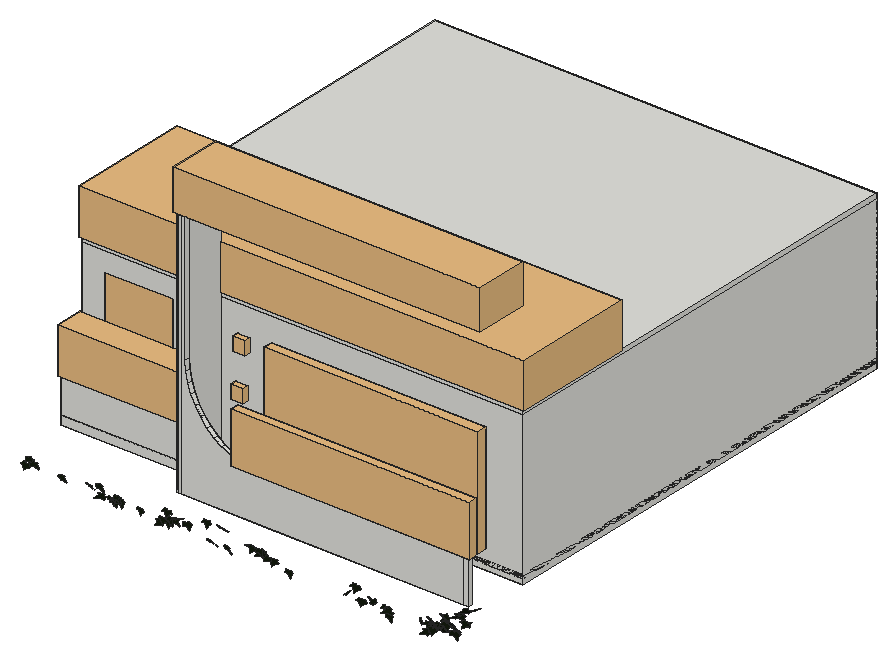
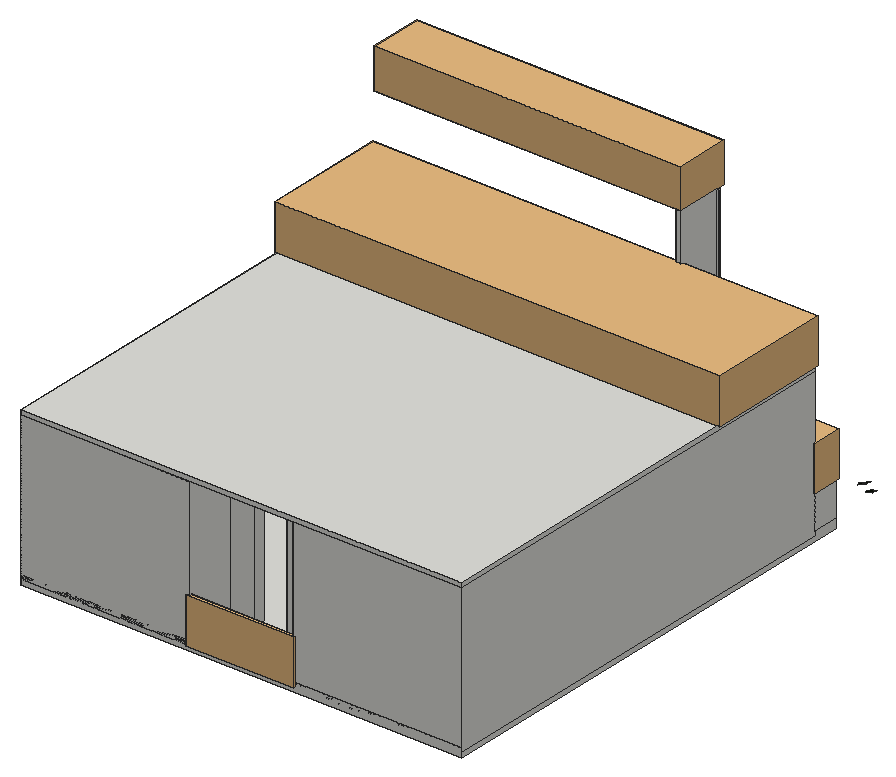
# SketchUp Ruby script. Lengths in millimetres.
U = 1.mm
M = Sketchup.active_model
def pt(a) = Geom::Point3d.new(a.map { |v| v * U })
def face(e, loops, mat)
  f = e.add_face(loops[0].map { |a| pt(a) })
  loops[1..].each { |l| e.add_face(l.map { |a| pt(a) }).erase! }
  f.material = f.back_material = mat if mat
  f
end
# faces: each face lists its corners as indices into pts; further lists are holes
def faces(e, pts, list, mat = nil) = list.each { |f| face(e, (f[0].is_a?(Array) ? f : [f]).map { |l| l.map { |i| pts[i] } }, mat) }
# xy, xz, yz: faces in a plane at the given z, y or x. An outline is a flat list of corners, or four numbers for a rectangle; further outlines are holes
def ring(l) = l.size == 4 ? [[l[0], l[1]], [l[2], l[1]], [l[2], l[3]], [l[0], l[3]]] : l.each_slice(2).to_a
def flat(e, list, mat, &to3) = list.each { |f| face(e, (f[0].is_a?(Array) ? f : [f]).map { |l| ring(l).map { |u, v| to3.(u, v) } }, mat) }
def xy(e, z, list, mat = nil) = flat(e, list, mat) { |x, y| [x, y, z] }
def xz(e, y, list, mat = nil) = flat(e, list, mat) { |x, z| [x, y, z] }
def yz(e, x, list, mat = nil) = flat(e, list, mat) { |y, z| [x, y, z] }
def lines(e, pts, list) = list.each { |a, b| e.add_line(pt(pts[a]), pt(pts[b])) }
# prism: a flat outline (further loops are holes) pulled along v
def prism(e, loops, v, mat = nil)
  f = face(e, loops, mat); d = Geom::Vector3d.new(v.map { |x| x * U })
  f.pushpull(f.normal.samedirection?(d) ? d.length : -d.length)
end
def box(e, o, s, mat = nil) = prism(e, [[o, [o[0] + s[0], o[1], o[2]], [o[0] + s[0], o[1] + s[1], o[2]], [o[0], o[1] + s[1], o[2]]]], [0, 0, s[2]], mat)
def at(x, y, z, deg = 0) = Geom::Transformation.translation(pt([x, y, z])) * Geom::Transformation.rotation(ORIGIN, Z_AXIS, deg.degrees)
def axes(o, x, y, z) = Geom::Transformation.new([*x, 0, *y, 0, *z, 0, *pt(o).to_a, 1])
def part(name) = M.definitions.add(name)
# library, detail: a bought-in or finely detailed component or shape, given as its bounding box
def library(name, o, s) = part(name).tap { |d| box(d.entities, o, s) }
def detail(e, o, s) = box(e.add_group.entities, o, s)
def put(e, d, t, mat = nil) = e.add_instance(d, t).tap { |i| i.material = mat if mat }
def group(e, t, mat = nil) = e.add_group.tap { |g| g.transformation = t; g.material = mat if mat }.entities
root = M.entities
M.materials.add("Emissive\#2").color = [255, 185, 108]
M.materials.add("efeu1").color = [18, 25, 13]
c1 = part("ivyleaf_9")
p = [[39.1,54.8,31.7],[34.5,51.8,30.2],[-5.3,25.2,17.3],[-17.9,28.3,20.9],[-21.6,21.7,17],[-20.2,4.3,5.3],
  [-22.9,-0.3,2.5],[-17.1,-4,-0.6],[-2,-2.1,-1.2],[-0.7,-15.4,-10.1],[16.6,-22.3,-16.7],[21.1,-15.1,-12.5],
  [32.7,-10.7,-11],[46.1,-1.8,-6.6],[30.8,11.2,3.8]]
faces(c1.entities,p,[[0,1,2,3,4,5,6,7,8,9,10,11,12,13,14]],"efeu1")
c2 = part("Group\#8")
g1 = group(c2.entities,at(0,0,0))
xy(g1,0,[[0,0,0,9144,3500.3,9144,3500.3,8102.6,4459.1,8102.6,4459.1,7874,3276.6,7874,3276.6,8915.4,228.6,8915.4,228.6,228.6,8915.4,228.6,8915.4,8915.4,5867.4,8915.4,5867.4,7874,5119.1,7874,5119.1,8102.6,5638.8,8102.6,5638.8,9144,9144,9144,9144,0]])
xy(g1,288,[[3929.6,0,8374.6,228.6],[4394.2,228.6,4521.2,579.4]])
xy(g1,376.3,[[475.3,0,1877,723.9]])
xy(g1,2564.5,[[3929.6,0,8374.6,228.6],[4394.2,228.6,4521.2,579.4]])
xy(g1,2644.4,[[475.3,0,1877,723.9]])
xy(g1,3048,[[0,0,9144,0,9144,9144,5638.8,9144,5638.8,8102.6,5119.1,8102.6,5119.1,7874,5867.4,7874,5867.4,8915.4,8915.4,8915.4,8915.4,228.6,228.6,228.6,228.6,8915.4,3276.6,8915.4,3276.6,7874,4459.1,7874,4459.1,8102.6,3500.3,8102.6,3500.3,9144,0,9144]])
xz(g1,0,[[[0,0,9144,3048],[3929.6,288,8374.6,2564.5],[475.3,376.3,1877,2644.4]]])
xz(g1,228.6,[[1447.8,0,1574.8,3048],[4394.2,0,4521.2,288],[4521.2,0,4521.2,288,8374.6,288,8374.6,2564.5,4521.2,2564.5,4521.2,3048,8915.4,3048,8915.4,0],[3929.6,288,4394.2,2564.5],[4394.2,2564.5,4521.2,3048]])
xz(g1,579.4,[[4394.2,288,4521.2,2564.5]])
xz(g1,723.9,[[475.3,376.3,1877,2644.4]])
xz(g1,7874,[[3276.6,0,3403.6,3048],[3403.6,0,4459.1,3048],[5119.1,0,5740.4,3048],[5740.4,0,5867.4,3048]])
xz(g1,8102.6,[[3500.3,0,4459.1,3048],[5119.1,0,5638.8,3048]])
xz(g1,8915.4,[[228.6,0,3276.6,3048],[5867.4,0,8915.4,3048]])
xz(g1,9144,[[0,0,3500.3,3048],[5638.8,0,9144,3048]])
yz(g1,0,[[0,0,9144,3048]])
yz(g1,228.6,[[228.6,0,2362.2,3048],[2362.2,0,2489.2,3048],[2489.2,0,5334,3048],[5334,0,5461,3048],[5461,0,8915.4,3048]])
yz(g1,475.3,[[0,376.3,723.9,2644.4]])
yz(g1,1877,[[0,376.3,723.9,2644.4]])
yz(g1,3276.6,[[7874,0,8915.4,3048]])
yz(g1,3500.3,[[8102.6,0,9144,3048]])
yz(g1,3929.6,[[0,288,228.6,2564.5]])
yz(g1,4394.2,[[228.6,288,579.4,2564.5]])
yz(g1,4459.1,[[7874,0,8102.6,3048]])
yz(g1,4521.2,[[228.6,288,579.4,2564.5]])
yz(g1,5119.1,[[7874,0,8102.6,3048]])
yz(g1,5638.8,[[8102.6,0,9144,3048]])
yz(g1,5867.4,[[7874,0,8915.4,3048]])
yz(g1,8374.6,[[0,288,228.6,2564.5]])
yz(g1,8915.4,[[228.6,0,5334,3048],[5334,0,5461,3048],[5461,0,8915.4,3048]])
yz(g1,9144,[[0,0,9144,3048]])
c3 = library("Group\#24",[0,0,0],[2238.5,80,939.4])
c4 = library("EP Casement KUN43",[213.5,133.1,19],[2173.1,999.9,208])
c5 = library("ITDHP",[-33.4,-34.2,-15.9],[968.5,150,1668.6])
c6 = library("Group\#17",[0,0,0],[2782,637.9,939.4])
c7 = library("Group\#26",[0,0,0],[4943.1,178,1057.4])
c8 = library("Spot Light\#2",[-129.6,-129.6,-280.7],[259.2,259.2,280.7])
c9 = part("Group263\#1")
p = [[0,0,0],[0,0,-885.4],[-221.6,0,-885.4],[1442.9,-1423.4,0],[-1442.9,-1423.4,0],[1442.9,1423.4,0],
  [1442.9,0,0],[-1442.9,1423.4,0],[221.6,0,-885.4],[-1442.9,0,0],[0,0,-1433.1]]
lines(c9.entities,p,[[0,1],[1,2],[3,4],[5,6],[7,5],[1,8],[9,0],[0,6],[8,10],[4,9],[6,3],[2,10],
  [9,7]])
c10 = part("Rectangle Light\#7")
put(c10.entities,c9,at(0,0,0))
c11 = library("Spot Light\#1",[-129.6,-129.6,-280.7],[259.2,259.2,280.7])
c12 = part("Group265\#1")
p = [[0,0,0],[0,0,-130.3],[-40.5,0,-130.3],[263.6,-158.2,0],[-263.6,-158.2,0],[263.6,158.2,0],
  [263.6,0,0],[-263.6,158.2,0],[40.5,0,-130.3],[-263.6,0,0],[0,0,-210.9]]
lines(c12.entities,p,[[0,1],[1,2],[3,4],[5,6],[7,5],[1,8],[9,0],[0,6],[8,10],[4,9],[6,3],[2,10],
  [9,7]])
c13 = part("Rectangle Light\#8")
put(c13.entities,c12,at(0,0,0))
c14 = part("Group267\#1")
p = [[0,0,0],[0,0,-108.5],[-7.2,0,-108.5],[46.9,-304.4,0],[-46.9,-304.4,0],[46.9,304.4,0],
  [46.9,0,0],[-46.9,304.4,0],[7.2,0,-108.5],[-46.9,0,0],[0,0,-175.7]]
lines(c14.entities,p,[[0,1],[1,2],[3,4],[5,6],[7,5],[1,8],[9,0],[0,6],[8,10],[4,9],[6,3],[2,10],
  [9,7]])
c15 = part("Rectangle Light\#9")
put(c15.entities,c14,at(0,0,0))
c16 = part("Group\#23")
box(c16.entities,[0,0,0],[9144,9144,101.6])
c17 = library("Group\#22",[0,0,0],[9224,2553.9,939.4])
c18 = library("Group\#21",[0,0,0],[6357.6,1104,823.9])
put(root,c1,axes([5592.3,460.8,6161.6],[2.45685,-0.59225,0.48479],[0.84867,-0.19058,-1.42023],[1.18387,1.3657,0.01204]))
put(root,c1,axes([4619,464.9,6158.3],[-2.79662,0.20864,-0.05049],[0.09953,0.00914,-1.48408],[-0.39623,-1.47027,-0.01639]))
put(root,c1,axes([10268,425.7,6170.1],[-1.4631,-1.24601,-0.25563],[0.22649,0.22692,-1.46397],[2.41017,-0.77771,-0.01761]))
put(root,c1,axes([7263.1,462.9,6167.7],[-0.14093,-1.51309,0.00427],[-0.04602,-0.00309,-1.51471],[2.87935,-0.07411,-0.024]))
put(root,c1,axes([4716.1,516.7,6171.9],[-0.7949,-1.4134,0.1654],[0.47802,-0.24289,-1.44133],[2.66582,-0.3779,0.30777]))
put(root,c1,axes([10372.8,511.1,6164.8],[1.65053,-0.29109,1.18272],[2.16594,-0.32374,-0.91416],[0.82609,1.43043,0.03378]))
put(root,c1,axes([10269.6,291.9,6174.6],[-2.74592,0.3863,0.12497],[-0.24273,0.00675,-1.49338],[-0.73361,-1.44818,0.02637]))
put(root,c1,axes([3627.4,500.3,6194.9],[-1.06639,-1.24057,-0.64669],[0.46448,0.59927,-1.36106],[2.62177,-0.61076,-0.02191]))
put(root,c1,axes([8473.7,494.3,6187.5],[-1.19113,1.32112,-0.36173],[0.25067,-0.33782,-1.46166],[-2.59482,-0.63908,0.02485]))
put(root,c1,axes([9436.4,340.7,6172.9],[0.14762,-1.48528,-0.01857],[-0.00283,0.01852,-1.4873],[2.827,0.07758,-0.00052]))
put(root,c1,axes([8823.4,415.7,6193.8],[-2.34891,-0.65133,-0.55971],[1.00163,0.20073,-1.39408],[1.29154,-1.34023,0.06322]))
put(root,c1,axes([1750.2,554.6,6179.2],[-1.73355,-1.13881,0.03125],[-0.03879,-0.02372,-1.45827],[2.16785,-0.91109,-0.0011]))
put(root,c1,axes([10180.6,478.7,6189.5],[2.52486,-0.3914,0.50724],[1.00699,0.01154,-1.37491],[0.68762,1.42026,0.15096]))
put(root,c1,axes([10669.4,492.6,6209.1],[-1.53123,-0.68677,-1.08449],[1.55876,0.71089,-1.05779],[1.88117,-1.14807,-0.00625]))
put(root,c1,axes([9258.6,483.9,6194.2],[-0.71663,-1.45468,-0.11155],[0.03481,0.11049,-1.50259],[2.77646,-0.37685,-0.00995]))
put(root,c1,axes([6901.1,527.6,6212.4],[-2.33936,-0.72135,-0.37924],[0.61848,0.19554,-1.4252],[1.4224,-1.2714,-0.00403]))
put(root,c1,axes([10275.7,523.5,6224],[1.15166,-1.06105,-0.84161],[-0.7576,0.74174,-1.22134],[2.46366,0.72409,0.01784]))
put(root,c1,axes([9997.1,453.2,6220.6],[1.22078,-0.32697,-1.31555],[-1.94024,0.8429,-0.70657],[1.70043,1.19651,0.13825]))
put(root,c1,axes([10372.5,513.3,6206.3],[-1.98775,1.05541,-0.06008],[0.05793,-0.0544,-1.48474],[-2.01108,-1.04474,0.01661]))
put(root,c1,axes([3561.3,487.2,6213.5],[0.11986,-1.46571,0.35331],[0.14084,-0.35019,-1.46594],[2.86597,0.07851,0.05726]))
put(root,c1,axes([10155.9,478.2,6205.5],[-1.17879,-1.33704,0.0176],[-0.02173,-0.0141,-1.47353],[2.54479,-0.61946,-0.00443]))
put(root,c1,axes([3736.6,494.1,6224.2],[-0.60958,-1.40382,-0.44375],[0.24382,0.42583,-1.4396],[2.79142,-0.34376,0.02884]))
put(root,c1,axes([2486.8,523.6,6229],[1.16186,-1.22558,-0.56432],[-0.00212,0.61894,-1.3454],[2.56791,0.55503,0.25422]))
put(root,c1,axes([4161.4,487.7,6217.2],[-0.35936,-1.3491,0.65494],[0.1835,-0.66966,-1.35163],[2.84826,-0.12707,0.16971]))
put(root,c1,axes([4630.4,482.4,6217.6],[-0.54586,-1.41103,0.41049],[0.0843,-0.42634,-1.43459],[2.79554,-0.26266,0.12341]))
put(root,c1,axes([6025.6,392.6,6215.5],[1.17613,-1.38471,0.05444],[0.03392,-0.05166,-1.51634],[2.63719,0.61822,-0.00478]))
put(root,c1,axes([9008.2,469.4,6194.5],[-0.34678,0.4928,1.41934],[-1.29932,1.24646,-0.52041],[-2.54723,-0.7029,0.07223]))
put(root,c1,axes([10409.4,951,6249.6],[-0.83955,-0.7574,-1.2019],[1.7959,0.78456,-0.84074],[2.02115,-1.01174,0.2478]))
put(root,c1,axes([6789.8,499.5,6240.5],[-1.69721,-0.94294,0.75948],[-0.06872,-0.92212,-1.18726],[2.30329,-0.72233,0.52421]))
put(root,c1,axes([9453.6,348.6,6241.1],[-2.38252,-0.35015,0.73544],[-1.15559,-0.49772,-1.27051],[1.03335,-1.36391,0.27483]))
put(root,c1,axes([4789.2,504.7,6251.5],[-0.70683,-1.42641,-0.28886],[0.04876,0.29167,-1.47319],[2.76942,-0.36919,-0.04779]))
put(root,c1,axes([1890.8,531.5,6266.3],[0.35247,-1.18685,-0.84705],[0.73603,0.86326,-1.125],[2.6757,-0.08112,0.42105]))
put(root,c1,axes([4809.8,510.3,6251.9],[-1.89205,-1.10921,0.08797],[0.2323,-0.22597,-1.46984],[2.1049,-0.97211,0.24129]))
put(root,c1,axes([3467.3,391.1,6258.1],[-2.76338,-0.00649,0.40098],[-0.76319,0.04278,-1.45134],[-0.00978,-1.50571,-0.04296]))
put(root,c1,axes([10436.3,963.2,6256.3],[-0.01243,1.47025,0.19647],[-0.16686,0.19574,-1.46774],[-2.81811,-0.01808,0.08604]))
put(root,c1,axes([4872,497.4,6274.7],[0.54961,-1.3483,-0.57095],[0.00487,0.58241,-1.37407],[2.78666,0.26491,0.11501]))
put(root,c1,axes([3669.7,492.1,6272.8],[0.37008,-1.48559,-0.22501],[0.23777,0.24209,-1.49037],[2.84971,0.17273,0.15357]))
g2 = group(root,at(1385.3,2446,6197.6))
xy(g2,0,[[[1.6,-547.9,1.6,9144,9144,9144,9144,0,2496.5,0,2496.5,-547.9],[313.2,-413.3,353.1,-408,390.2,-392.6,422.1,-368.2,446.6,-336.3,462,-299.1,467.2,-259.3,462,-219.4,446.6,-182.3,422.1,-150.4,390.2,-125.9,353.1,-110.5,313.2,-105.3,273.4,-110.5,236.2,-125.9,204.3,-150.4,179.9,-182.3,164.5,-219.4,159.2,-259.3,164.5,-299.1,179.9,-336.3,204.3,-368.2,236.2,-392.6,273.4,-408],[1249,-413.3,1288.9,-408,1326,-392.6,1357.9,-368.2,1382.4,-336.3,1397.8,-299.1,1403,-259.3,1397.8,-219.4,1382.4,-182.3,1357.9,-150.4,1326,-125.9,1288.9,-110.5,1249,-105.3,1209.2,-110.5,1172.1,-125.9,1140.2,-150.4,1115.7,-182.3,1100.3,-219.4,1095.1,-259.3,1100.3,-299.1,1115.7,-336.3,1140.2,-368.2,1172.1,-392.6,1209.2,-408],[2184.9,-413.3,2224.7,-408,2261.9,-392.6,2293.8,-368.2,2318.2,-336.3,2333.6,-299.1,2338.9,-259.3,2333.6,-219.4,2318.2,-182.3,2293.8,-150.4,2261.9,-125.9,2224.7,-110.5,2184.9,-105.3,2145,-110.5,2107.9,-125.9,2076,-150.4,2051.5,-182.3,2036.1,-219.4,2030.9,-259.3,2036.1,-299.1,2051.5,-336.3,2076,-368.2,2107.9,-392.6,2145,-408]],[[313.2,-413.3,273.4,-408,236.2,-392.6,204.3,-368.2,179.9,-336.3,164.5,-299.1,159.2,-259.3,164.5,-219.4,179.9,-182.3,204.3,-150.4,236.2,-125.9,273.4,-110.5,313.2,-105.3,353.1,-110.5,390.2,-125.9,422.1,-150.4,446.6,-182.3,462,-219.4,467.2,-259.3,462,-299.1,446.6,-336.3,422.1,-368.2,390.2,-392.6,353.1,-408],[313.2,-357.7,338.7,-354.4,362.4,-344.5,382.8,-328.9,398.5,-308.5,408.3,-284.8,411.6,-259.3,408.3,-233.8,398.5,-210.1,382.8,-189.7,362.4,-174,338.7,-164.2,313.2,-160.9,287.7,-164.2,264,-174,243.6,-189.7,228,-210.1,218.1,-233.8,214.8,-259.3,218.1,-284.8,228,-308.5,243.6,-328.9,264,-344.5,287.7,-354.4]],[[1249,-413.3,1209.2,-408,1172.1,-392.6,1140.2,-368.2,1115.7,-336.3,1100.3,-299.1,1095.1,-259.3,1100.3,-219.4,1115.7,-182.3,1140.2,-150.4,1172.1,-125.9,1209.2,-110.5,1249,-105.3,1288.9,-110.5,1326,-125.9,1357.9,-150.4,1382.4,-182.3,1397.8,-219.4,1403,-259.3,1397.8,-299.1,1382.4,-336.3,1357.9,-368.2,1326,-392.6,1288.9,-408],[1249,-357.7,1274.5,-354.4,1298.3,-344.5,1318.6,-328.9,1334.3,-308.5,1344.1,-284.8,1347.5,-259.3,1344.1,-233.8,1334.3,-210.1,1318.6,-189.7,1298.3,-174,1274.5,-164.2,1249,-160.9,1223.6,-164.2,1199.8,-174,1179.5,-189.7,1163.8,-210.1,1154,-233.8,1150.6,-259.3,1154,-284.8,1163.8,-308.5,1179.5,-328.9,1199.8,-344.5,1223.6,-354.4]],[[2184.9,-413.3,2145,-408,2107.9,-392.6,2076,-368.2,2051.5,-336.3,2036.1,-299.1,2030.9,-259.3,2036.1,-219.4,2051.5,-182.3,2076,-150.4,2107.9,-125.9,2145,-110.5,2184.9,-105.3,2224.7,-110.5,2261.9,-125.9,2293.8,-150.4,2318.2,-182.3,2333.6,-219.4,2338.9,-259.3,2333.6,-299.1,2318.2,-336.3,2293.8,-368.2,2261.9,-392.6,2224.7,-408],[2184.9,-357.7,2210.4,-354.4,2234.1,-344.5,2254.5,-328.9,2270.1,-308.5,2280,-284.8,2283.3,-259.3,2280,-233.8,2270.1,-210.1,2254.5,-189.7,2234.1,-174,2210.4,-164.2,2184.9,-160.9,2159.4,-164.2,2135.7,-174,2115.3,-189.7,2099.6,-210.1,2089.8,-233.8,2086.5,-259.3,2089.8,-284.8,2099.6,-308.5,2115.3,-328.9,2135.7,-344.5,2159.4,-354.4]]])
xy(g2,46,[[313.2,-357.7,287.7,-354.4,264,-344.5,243.6,-328.9,228,-308.5,218.1,-284.8,214.8,-259.3,218.1,-233.8,228,-210.1,243.6,-189.7,264,-174,287.7,-164.2,313.2,-160.9,338.7,-164.2,362.4,-174,382.8,-189.7,398.5,-210.1,408.3,-233.8,411.6,-259.3,408.3,-284.8,398.5,-308.5,382.8,-328.9,362.4,-344.5,338.7,-354.4],[1249,-357.7,1223.6,-354.4,1199.8,-344.5,1179.5,-328.9,1163.8,-308.5,1154,-284.8,1150.6,-259.3,1154,-233.8,1163.8,-210.1,1179.5,-189.7,1199.8,-174,1223.6,-164.2,1249,-160.9,1274.5,-164.2,1298.3,-174,1318.6,-189.7,1334.3,-210.1,1344.1,-233.8,1347.5,-259.3,1344.1,-284.8,1334.3,-308.5,1318.6,-328.9,1298.3,-344.5,1274.5,-354.4],[2184.9,-357.7,2159.4,-354.4,2135.7,-344.5,2115.3,-328.9,2099.6,-308.5,2089.8,-284.8,2086.5,-259.3,2089.8,-233.8,2099.6,-210.1,2115.3,-189.7,2135.7,-174,2159.4,-164.2,2184.9,-160.9,2210.4,-164.2,2234.1,-174,2254.5,-189.7,2270.1,-210.1,2280,-233.8,2283.3,-259.3,2280,-284.8,2270.1,-308.5,2254.5,-328.9,2234.1,-344.5,2210.4,-354.4]],"Emissive\#2")
xy(g2,188.9,[[1.6,-547.9,2496.5,-547.9,2496.5,0,9144,0,9144,9144,1.6,9144]])
xz(g2,-547.9,[[1.6,0,2496.5,188.9]])
xz(g2,0,[[2496.5,0,9144,188.9]])
xz(g2,9144,[[1.6,0,9144,188.9]])
yz(g2,1.6,[[-547.9,0,9144,188.9]])
yz(g2,2496.5,[[-547.9,0,0,188.9]])
yz(g2,9144,[[0,0,9144,188.9]])
p = [[313.2,-357.7,0],[287.7,-354.4,0],[287.7,-354.4,46],[313.2,-357.7,46],[338.7,-354.4,0],[338.7,-354.4,46],
  [1249,-357.7,0],[1223.6,-354.4,0],[1223.6,-354.4,46],[1249,-357.7,46],[1274.5,-354.4,0],[1274.5,-354.4,46],
  [2184.9,-357.7,0],[2159.4,-354.4,0],[2159.4,-354.4,46],[2184.9,-357.7,46],[2210.4,-354.4,0],[2210.4,-354.4,46],
  [264,-344.5,0],[264,-344.5,46],[362.4,-344.5,0],[362.4,-344.5,46],[1199.8,-344.5,0],[1199.8,-344.5,46],
  [1298.3,-344.5,0],[1298.3,-344.5,46],[2135.7,-344.5,0],[2135.7,-344.5,46],[2234.1,-344.5,0],[2234.1,-344.5,46],
  [243.6,-328.9,0],[243.6,-328.9,46],[382.8,-328.9,0],[382.8,-328.9,46],[1179.5,-328.9,0],[1179.5,-328.9,46],
  [1318.6,-328.9,0],[1318.6,-328.9,46],[2115.3,-328.9,0],[2115.3,-328.9,46],[2254.5,-328.9,0],[2254.5,-328.9,46],
  [228,-308.5,0],[228,-308.5,46],[398.5,-308.5,0],[398.5,-308.5,46],[1163.8,-308.5,0],[1163.8,-308.5,46],
  [1334.3,-308.5,0],[1334.3,-308.5,46],[2099.6,-308.5,0],[2099.6,-308.5,46],[2270.1,-308.5,0],[2270.1,-308.5,46],
  [218.1,-284.8,0],[218.1,-284.8,46],[408.3,-284.8,0],[408.3,-284.8,46],[1154,-284.8,0],[1154,-284.8,46],
  [1344.1,-284.8,0],[1344.1,-284.8,46],[2089.8,-284.8,0],[2089.8,-284.8,46],[2280,-284.8,0],[2280,-284.8,46],
  [214.8,-259.3,0],[214.8,-259.3,46],[411.6,-259.3,0],[411.6,-259.3,46],[1150.6,-259.3,0],[1150.6,-259.3,46],
  [1347.5,-259.3,0],[1347.5,-259.3,46],[2086.5,-259.3,0],[2086.5,-259.3,46],[2283.3,-259.3,0],[2283.3,-259.3,46],
  [218.1,-233.8,0],[218.1,-233.8,46],[408.3,-233.8,0],[408.3,-233.8,46],[1154,-233.8,0],[1154,-233.8,46],
  [1344.1,-233.8,0],[1344.1,-233.8,46],[2089.8,-233.8,0],[2089.8,-233.8,46],[2280,-233.8,0],[2280,-233.8,46],
  [228,-210.1,0],[228,-210.1,46],[398.5,-210.1,0],[398.5,-210.1,46],[1163.8,-210.1,0],[1163.8,-210.1,46],
  [1334.3,-210.1,0],[1334.3,-210.1,46],[2099.6,-210.1,0],[2099.6,-210.1,46],[2270.1,-210.1,0],[2270.1,-210.1,46],
  [243.6,-189.7,0],[243.6,-189.7,46],[382.8,-189.7,0],[382.8,-189.7,46],[1179.5,-189.7,0],[1179.5,-189.7,46],
  [1318.6,-189.7,0],[1318.6,-189.7,46],[2115.3,-189.7,0],[2115.3,-189.7,46],[2254.5,-189.7,0],[2254.5,-189.7,46],
  [264,-174,0],[264,-174,46],[362.4,-174,0],[362.4,-174,46],[1199.8,-174,0],[1199.8,-174,46],
  [1298.3,-174,0],[1298.3,-174,46],[2135.7,-174,0],[2135.7,-174,46],[2234.1,-174,0],[2234.1,-174,46],
  [287.7,-164.2,0],[287.7,-164.2,46],[338.7,-164.2,0],[338.7,-164.2,46],[1223.6,-164.2,0],[1223.6,-164.2,46],
  [1274.5,-164.2,0],[1274.5,-164.2,46],[2159.4,-164.2,0],[2159.4,-164.2,46],[2210.4,-164.2,0],[2210.4,-164.2,46],
  [313.2,-160.9,0],[313.2,-160.9,46],[1249,-160.9,0],[1249,-160.9,46],[2184.9,-160.9,0],[2184.9,-160.9,46],
  [2496.5,0,-1.8],[2496.5,0,0]]
faces(g2,p,[[0,1,2,3],[4,0,3,5],[6,7,8,9],[10,6,9,11],[12,13,14,15],[16,12,15,17],[1,18,19,2],[20,4,5,21],
  [7,22,23,8],[24,10,11,25],[13,26,27,14],[28,16,17,29],[18,30,31,19],[32,20,21,33],[22,34,35,23],[36,24,25,37],
  [26,38,39,27],[40,28,29,41],[30,42,43,31],[44,32,33,45],[34,46,47,35],[48,36,37,49],[38,50,51,39],[52,40,41,53],
  [42,54,55,43],[56,44,45,57],[46,58,59,47],[60,48,49,61],[50,62,63,51],[64,52,53,65],[54,66,67,55],[68,56,57,69],
  [58,70,71,59],[72,60,61,73],[62,74,75,63],[76,64,65,77],[66,78,79,67],[80,68,69,81],[70,82,83,71],[84,72,73,85],
  [74,86,87,75],[88,76,77,89],[78,90,91,79],[92,80,81,93],[82,94,95,83],[96,84,85,97],[86,98,99,87],[100,88,89,101],
  [90,102,103,91],[104,92,93,105],[94,106,107,95],[108,96,97,109],[98,110,111,99],[112,100,101,113],[102,114,115,103],[116,104,105,117],
  [106,118,119,107],[120,108,109,121],[110,122,123,111],[124,112,113,125],[114,126,127,115],[128,116,117,129],[118,130,131,119],[132,120,121,133],
  [122,134,135,123],[136,124,125,137],[126,138,139,127],[138,128,129,139],[130,140,141,131],[140,132,133,141],[134,142,143,135],[142,136,137,143]],"Emissive\#2")
lines(g2,p,[[144,145]])
put(root,c1,axes([10492.7,508.2,6302.1],[-1.49498,-1.07711,-0.67774],[0.69889,0.57073,-1.33264],[2.31897,-0.86639,-0.03529]))
g3 = group(root,at(10529.3,1322.1,6197.6))
xy(g3,0,[[-6178.7,0,-4589,0,-4589,85.5,-6261.6,85.5,-6261.6,1124,-6377.5,1124,-6377.5,198.8,-6372,138.1,-6355.4,88.4,-6327.8,49.7,-6289.2,22.1,-6239.5,5.5],[-4589,0,-341.4,0,-237.1,9.5,-237.1,85.5,-4589,85.5]])
xy(g3,914.4,[[-4589,0,-4589,85.5,-237.1,85.5,-237.1,9.5,-341.4,0]])
xy(g3,5167.3,[[-6178.7,0,-6239.5,5.5,-6289.2,22.1,-6327.8,49.7,-6355.4,88.4,-6372,138.1,-6377.5,198.8,-6377.5,1124,-6261.6,1124,-6261.6,85.5,-6107.5,85.5,-6107.5,0]])
xz(g3,0,[[-6178.7,0,-6178.7,5167.3,-6107.5,5167.3,-6107.5,2515.5,-6089.7,2315.1,-6047.6,2118.3,-5981.9,1928.1,-5893.6,1747.3,-5784,1578.5,-5654.7,1424.4,-5507.6,1287.1,-5344.9,1168.7,-5169,1070.9,-4982.5,995.3,-4788.2,942.8,-4589,914.4,-341.4,914.4,-341.4,0]])
xz(g3,85.5,[[-6261.6,0,-4589,0,-4589,914.4,-4788.2,942.8,-4982.5,995.3,-5169,1070.9,-5344.9,1168.7,-5507.6,1287.1,-5654.7,1424.4,-5784,1578.5,-5893.6,1747.3,-5981.9,1928.1,-6047.6,2118.3,-6089.7,2315.1,-6107.5,2515.5,-6107.5,5167.3,-6261.6,5167.3],[-4589,0,-237.1,914.4]])
xz(g3,1124,[[-6377.5,0,-6261.6,5167.3]])
yz(g3,-6377.5,[[198.8,0,1124,5167.3]])
yz(g3,-6261.6,[[85.5,0,1124,5167.3]])
yz(g3,-6107.5,[[0,2515.5,85.5,5167.3]])
yz(g3,-237.1,[[9.5,0,85.5,914.4]])
p = [[-6239.5,5.5,0],[-6239.5,5.5,5167.3],[-6178.7,0,5167.3],[-6178.7,0,0],[-237.1,9.5,914.4],[-237.1,9.5,0],
  [-341.4,0,0],[-341.4,0,914.4],[-6289.2,22.1,0],[-6289.2,22.1,5167.3],[-6327.8,49.7,0],[-6327.8,49.7,5167.3],
  [-6355.4,88.4,0],[-6355.4,88.4,5167.3],[-6372,138.1,0],[-6372,138.1,5167.3],[-6377.5,198.8,0],[-6377.5,198.8,5167.3],
  [-4589,0,914.4],[-4788.2,0,942.8],[-4788.2,85.5,942.8],[-4589,85.5,914.4],[-4982.5,0,995.3],[-4982.5,85.5,995.3],
  [-5169,0,1070.9],[-5169,85.5,1070.9],[-5344.9,0,1168.7],[-5344.9,85.5,1168.7],[-5507.6,0,1287.1],[-5507.6,85.5,1287.1],
  [-5654.7,0,1424.4],[-5654.7,85.5,1424.4],[-5784,0,1578.5],[-5784,85.5,1578.5],[-5893.6,0,1747.3],[-5893.6,85.5,1747.3],
  [-5981.9,0,1928.1],[-5981.9,85.5,1928.1],[-6047.6,0,2118.3],[-6047.6,85.5,2118.3],[-6089.7,0,2315.1],[-6089.7,85.5,2315.1],
  [-6107.5,0,2515.5],[-6107.5,85.5,2515.5],[-237.1,85.5,0],[-166.7,85.5,0]]
faces(g3,p,[[0,1,2,3],[4,5,6,7],[8,9,1,0],[10,11,9,8],[12,13,11,10],[14,15,13,12],[16,17,15,14],[18,19,20,21],
  [19,22,23,20],[22,24,25,23],[24,26,27,25],[26,28,29,27],[28,30,31,29],[30,32,33,31],[32,34,35,33],[34,36,37,35],
  [36,38,39,37],[38,40,41,39],[40,42,43,41]])
lines(g3,p,[[44,45]])
put(root,c1,axes([10125.2,494.5,6295.2],[1.91891,-1.0814,0.05819],[0.48373,0.15901,-1.44897],[2.00354,0.99734,0.2941]))
put(root,c1,axes([1811.6,546.7,6312.7],[0.09495,-1.401,-0.45119],[0.32585,0.45391,-1.3905],[2.78222,-0.00535,0.17825]))
put(root,c1,axes([6355.4,512.7,6312.4],[2.60802,0.02019,0.57035],[1.03518,0.403,-1.32108],[-0.32889,1.42853,0.36463]))
put(root,c1,axes([6738.1,453.5,6319.9],[-2.70644,-0.23671,0.40812],[-0.77066,-0.05277,-1.44154],[0.46081,-1.47851,-0.01389]))
put(root,c1,axes([3107,481,6293.7],[2.444,-0.54338,-0.53235],[0.93724,-0.20228,1.39438],[-1.10345,-1.37533,0.00525]))
put(root,c1,axes([10652.9,454.3,6332],[2.36849,-0.84952,-0.07029],[0.33347,0.37665,-1.4501],[1.58769,1.18819,0.40942]))
put(root,c1,axes([6679.1,458.5,6352],[-0.66879,-1.36353,-0.56016],[0.33468,0.53297,-1.40766],[2.78549,-0.39142,0.03464]))
put(root,c1,axes([6535.4,460.3,6343.6],[-1.77797,-1.09073,0.49098],[0.11257,-0.66435,-1.36332],[2.27371,-0.82002,0.45143]))
put(root,c1,axes([4996.6,424.4,6359.3],[0.86145,1.4208,-0.19565],[-0.89305,-0.04716,-1.42808],[-2.57936,0.49085,0.4291]))
put(root,c1,axes([5214,378.2,6377.3],[-0.59788,-1.32015,-0.67244],[0.33084,0.6498,-1.35691],[2.8002,-0.35864,0.01674]))
put(root,c1,axes([10575.7,945.2,6392.5],[-0.47424,0.48957,-1.39508],[-0.47616,-1.40831,-0.44952],[-2.77327,0.15808,0.31575]))
put(root,c2,at(1385.3,2446,6299.2))
put(root,c3,at(4835.6,11550,6299.2))
put(root,c1,axes([10616.1,425.3,6400.7],[2.72641,-0.02176,-0.46209],[-0.87822,0.03915,-1.43238],[0.06228,1.50471,0.03058]))
put(root,c1,axes([3349.1,424.7,6409.6],[0.61234,-1.42081,-0.39279],[0.08673,0.41144,-1.45091],[2.80418,0.29753,0.13065]))
put(root,c1,axes([8689.6,421.4,6410.6],[-2.36553,-0.72594,-0.4531],[0.78809,0.18901,-1.43873],[1.42527,-1.30936,0.04353]))
put(root,c1,axes([10877.1,549.3,6423.1],[-2.76867,-0.33173,-0.21912],[0.41614,0.02661,-1.49192],[0.63194,-1.47091,0.02242]))
put(root,c1,axes([10935.7,542.1,6437.3],[-1.61362,1.15724,-0.48836],[0.25883,-0.50117,-1.42368],[-2.37649,-0.84034,0.17654]))
put(root,c1,axes([4770.5,434.6,6427.3],[-1.3502,-1.32986,0.06257],[-0.06448,-0.05284,-1.50725],[2.53297,-0.71023,-0.00502]))
put(root,c1,axes([10437.8,465,6456.8],[1.44524,-1.15284,0.62338],[0.7666,-0.48029,-1.3789],[2.37359,0.85707,0.06578]))
put(root,c1,axes([10735,958.6,6451.1],[0.66847,1.45728,0.12768],[0.06691,0.12286,-1.499],[-2.78332,0.35295,-0.00537]))
put(root,c1,axes([10542.4,463.8,6463.7],[-2.73291,0.34118,-0.2743],[0.50945,-0.05999,-1.47592],[-0.65926,-1.46069,-0.00345]))
put(root,c1,axes([5806.3,484.3,6468.2],[1.40047,-0.88931,0.97074],[1.69779,-0.48104,-1.11691],[1.84267,1.11911,0.29131]))
g4 = group(root,at(1385.3,1898.1,6387.3))
prism(g4,[[[2822.1,0,0],[0,0,0],[0,547.9,0],[93.2,547.9,0],[93.2,158.8,0],[2822.1,158.8,0]]],[0,0,724.7])
put(root,c1,axes([5565.4,455.3,6498.2],[-0.72201,-1.46477,0.04473],[-0.01268,-0.04448,-1.51309],[2.78902,-0.3794,0.0047]))
put(root,c1,axes([10744.6,419.7,6565.5],[0.88311,1.44174,0.03291],[-0.00779,0.03589,-1.5145],[-2.74463,0.46379,0.01489]))
put(root,c4,axes([4878.3,2465.1,6284.3],[2.04542,0,0],[0,0,2.2766],[0,-1,0]))
put(root,c5,axes([1909.4,2477.6,6697],[1.44679,0,0],[0,0.92467,0],[0,0,1.35933]))
put(root,c6,at(1345.3,1858.1,7112))
put(root,c7,at(5399.5,1282.1,7112))
put(root,c8,at(4699.8,2446,7886))
put(root,c10,at(7178.4,5912.8,9346.9))
put(root,c11,at(4733.8,2446,8790.9))
put(root,c13,at(2342.3,2937.7,8943.3))
put(root,c15,at(3107.3,2750.4,8943.3))
put(root,c16,at(1385.3,2446,9347.2))
put(root,c17,at(1345.3,2406,9448.8))
put(root,c18,at(4151.8,1342,11364.9))
